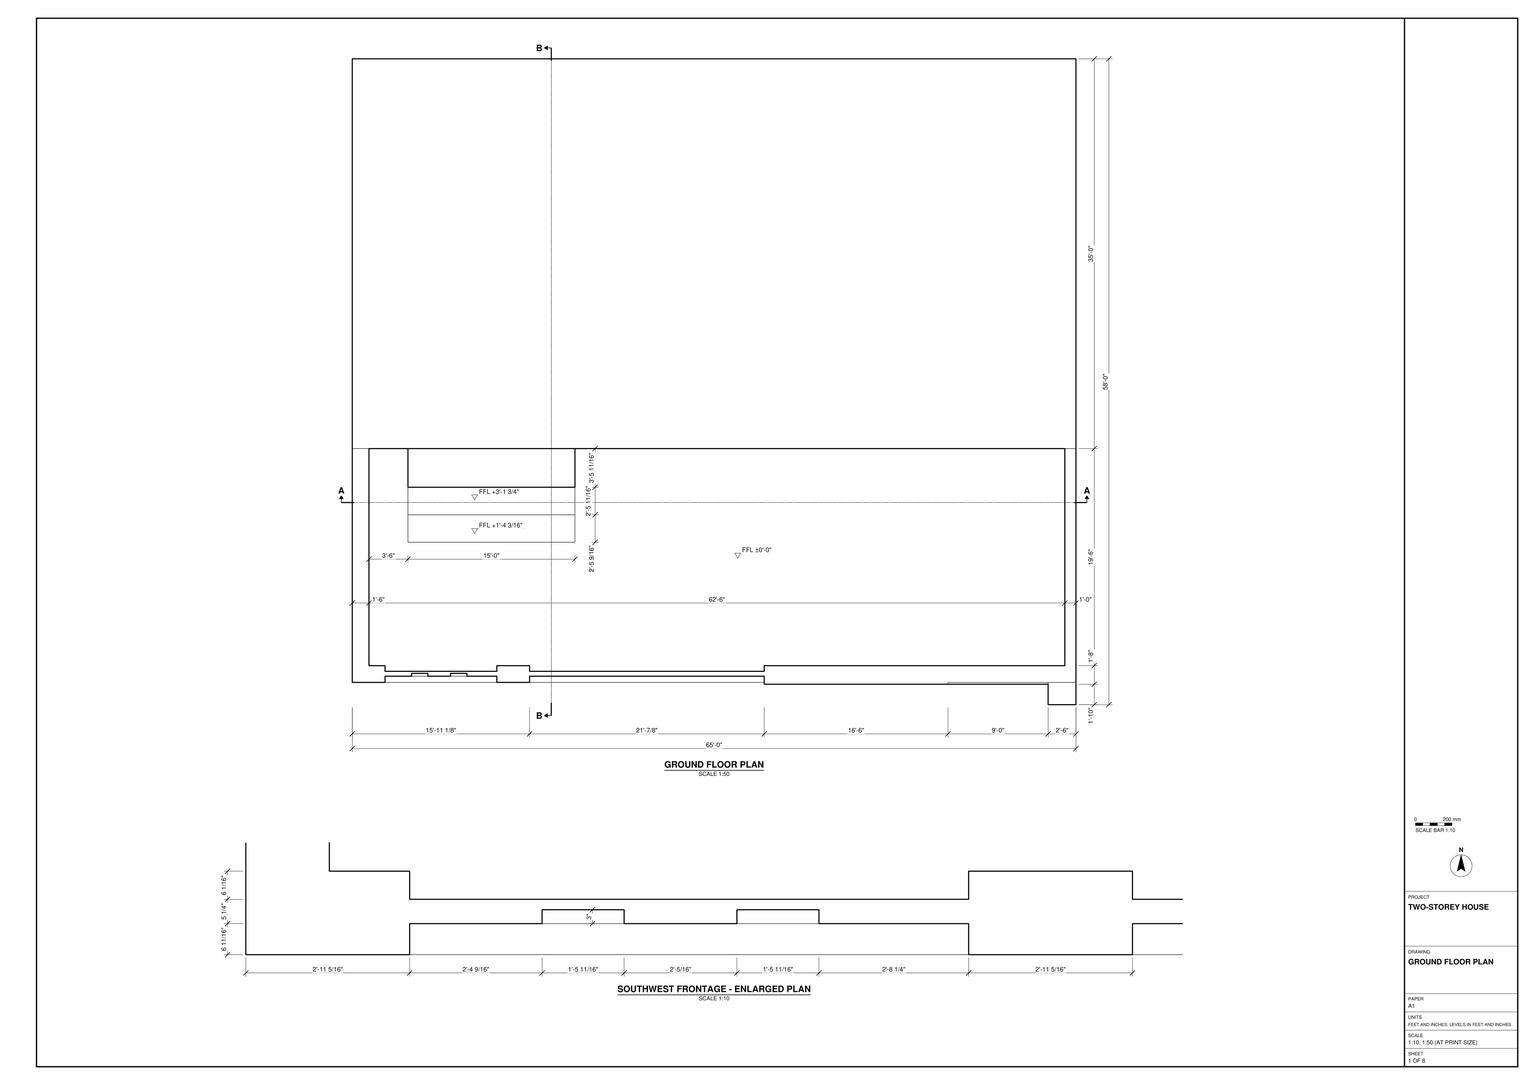
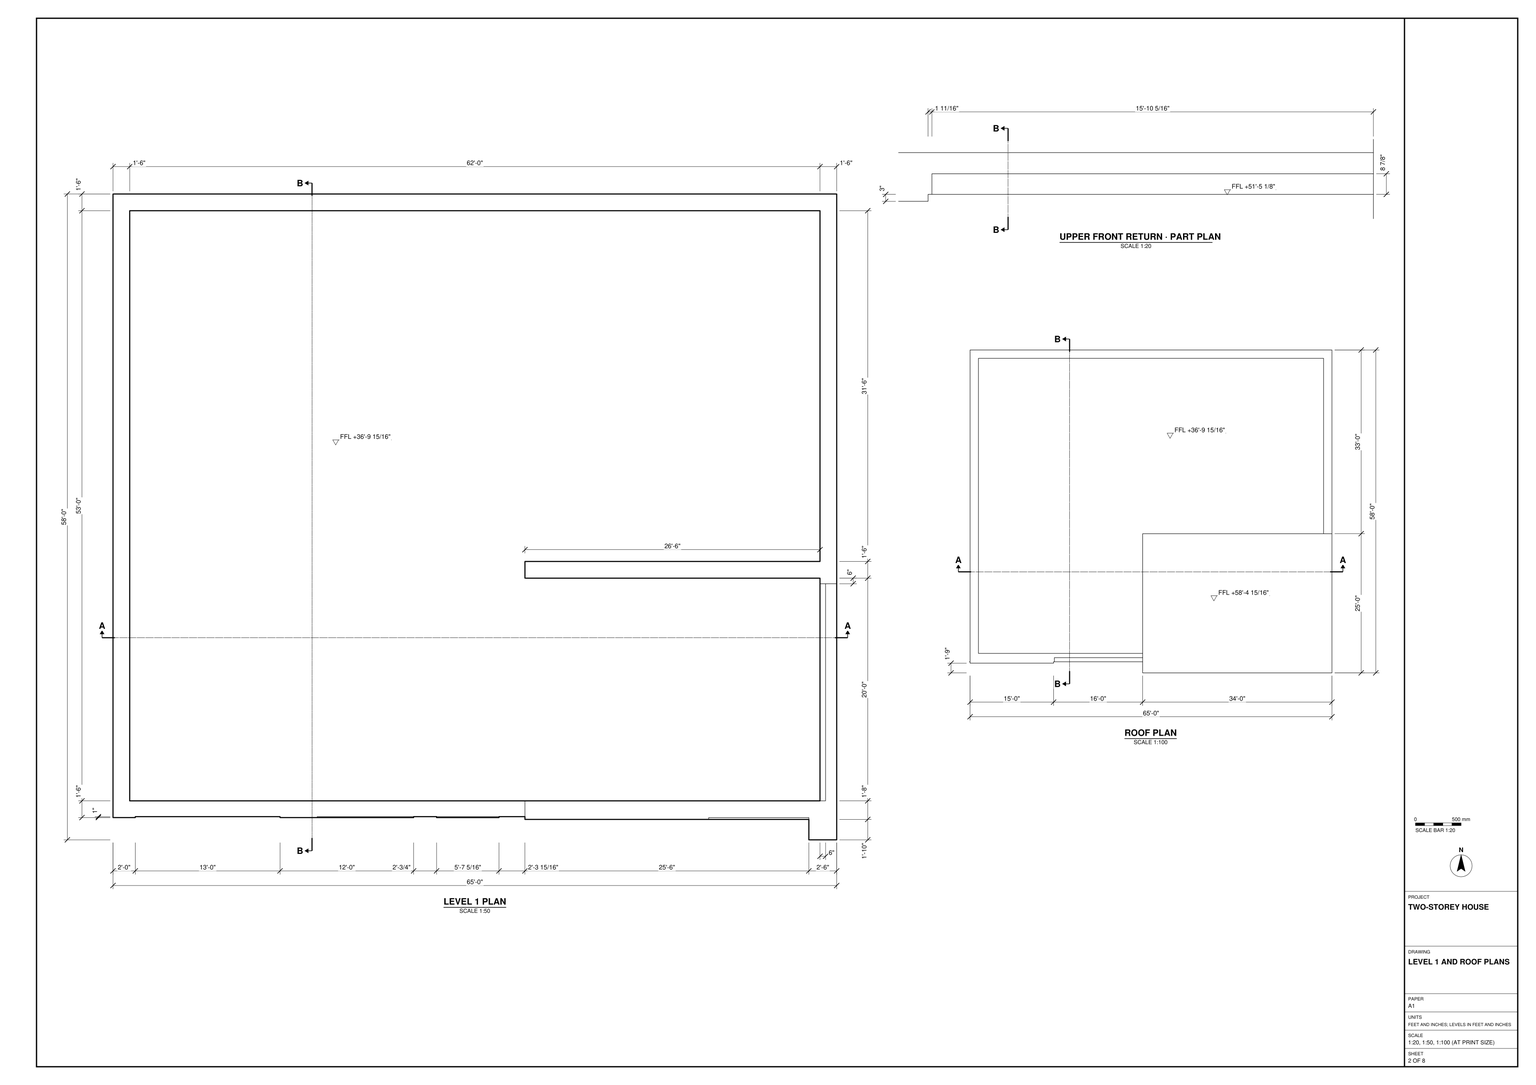
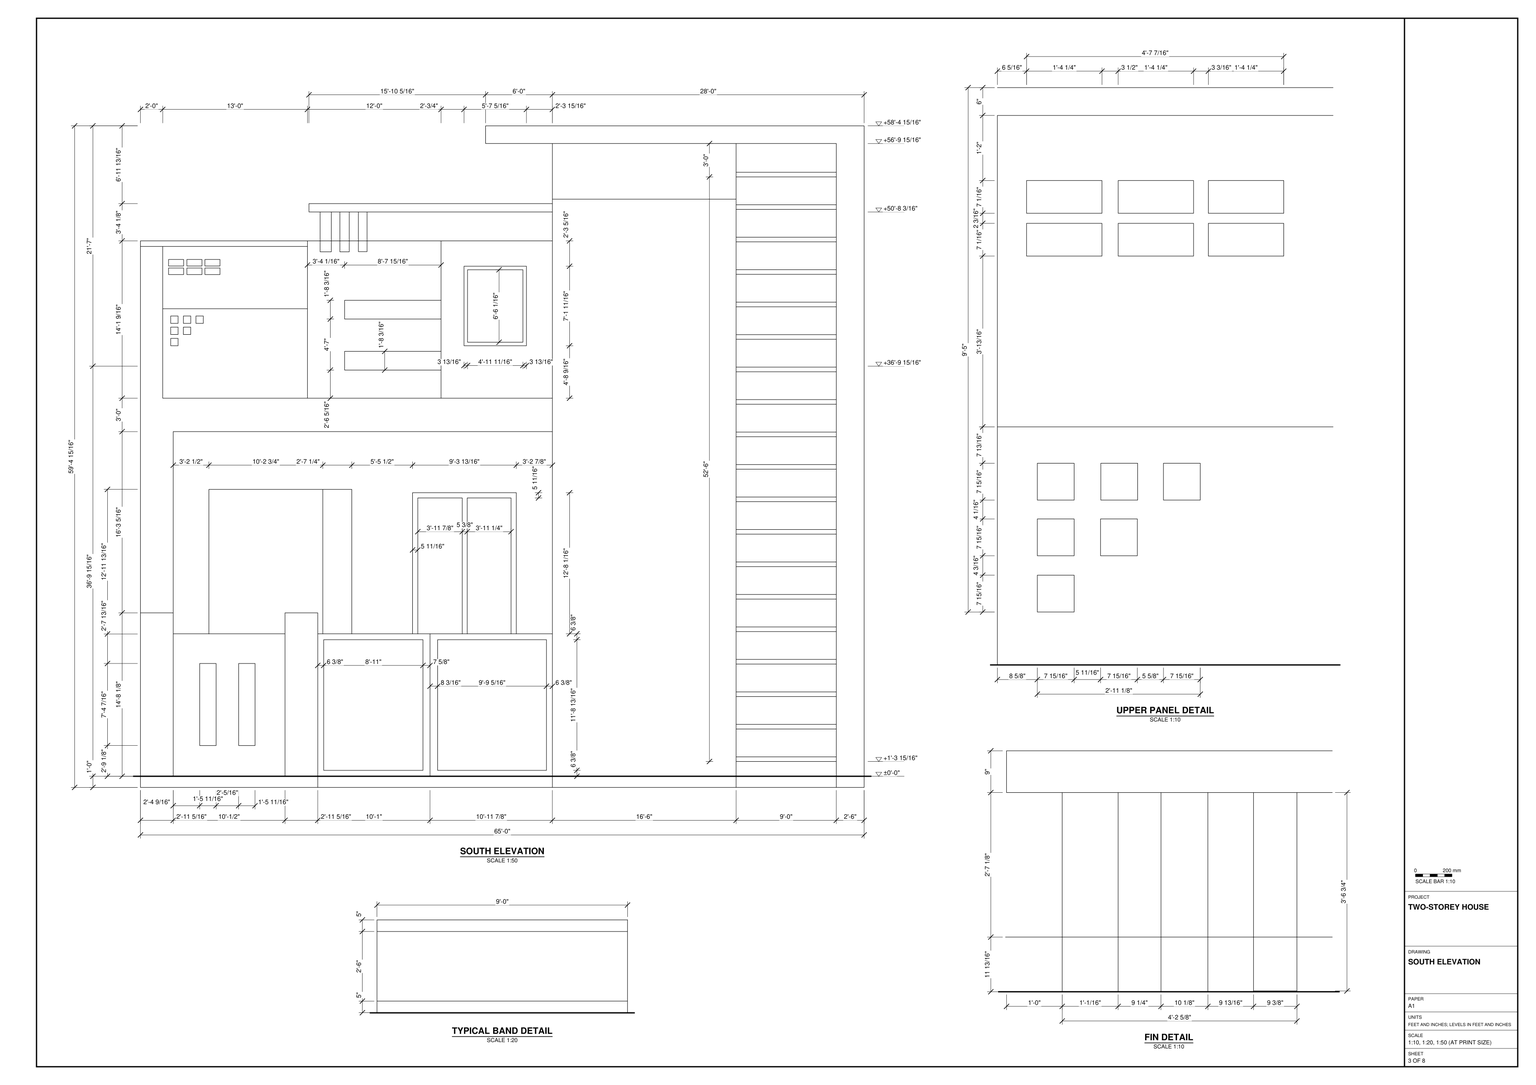
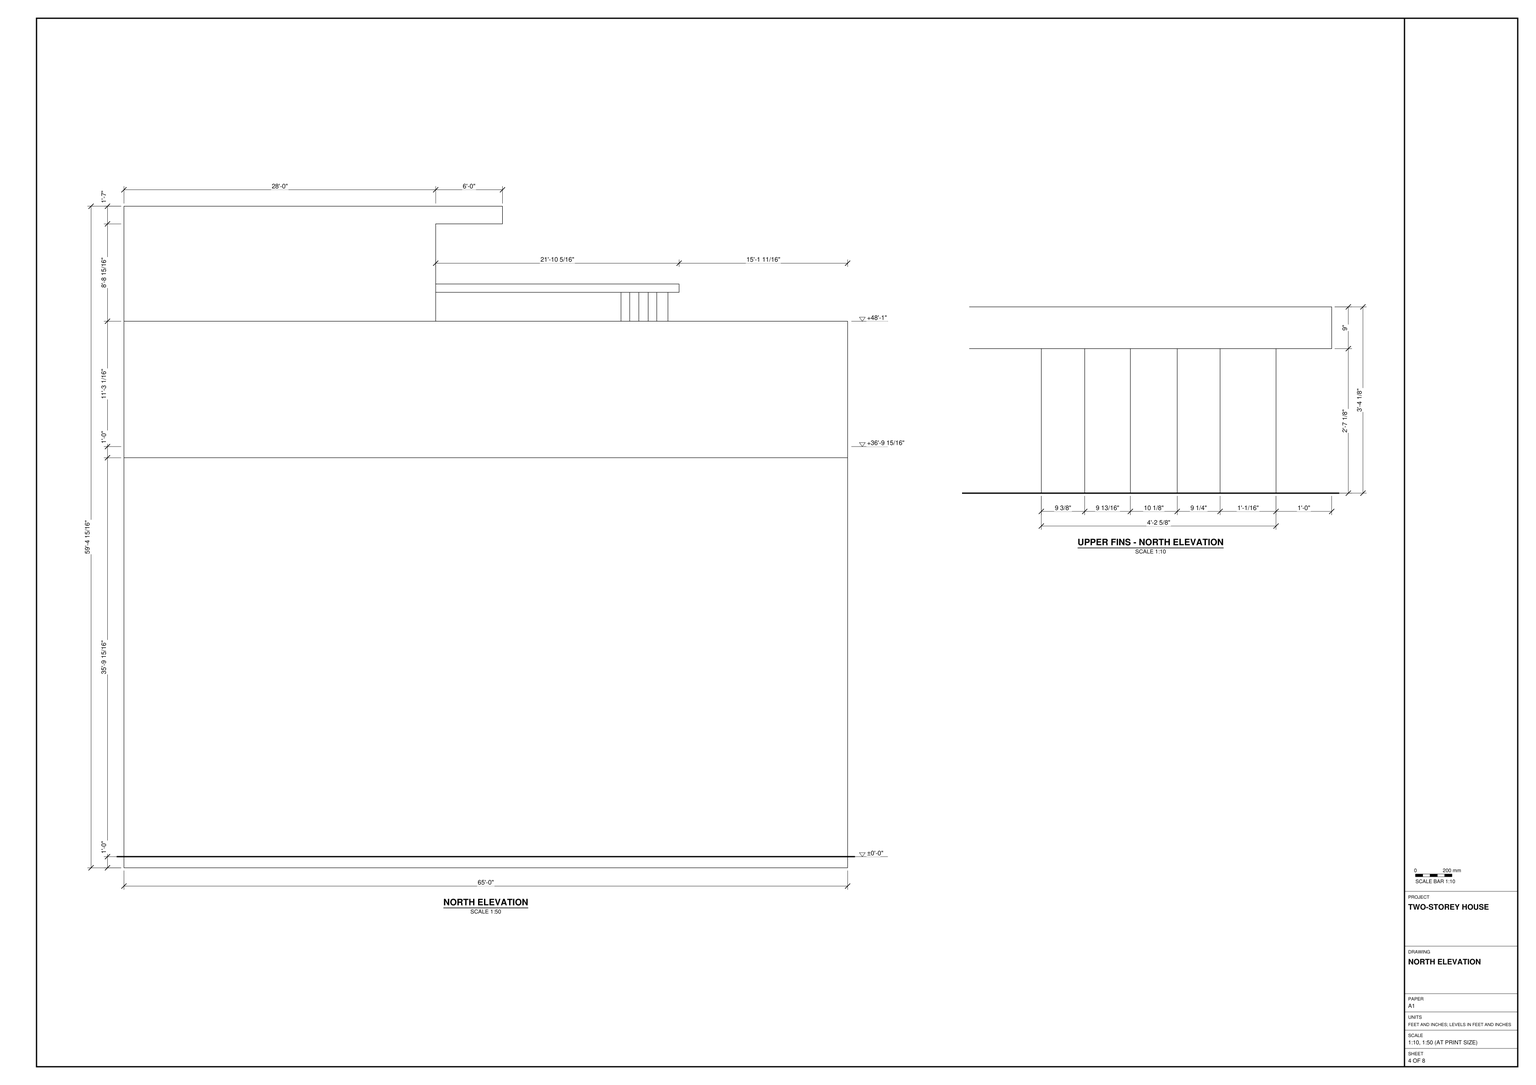
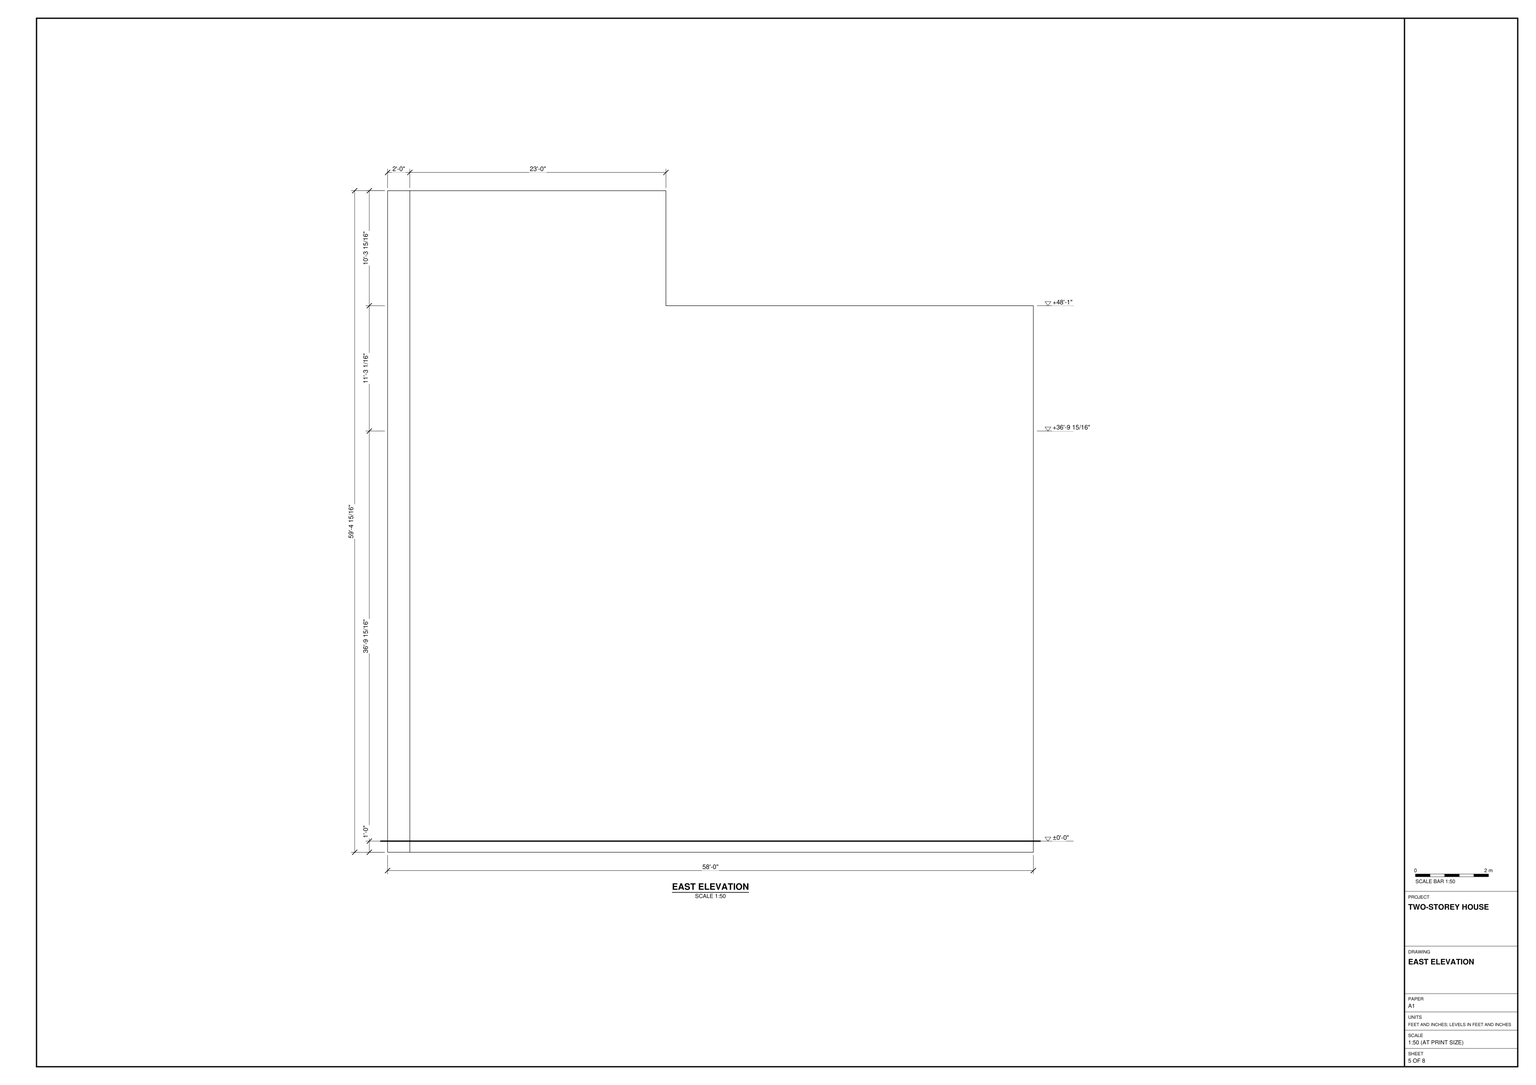
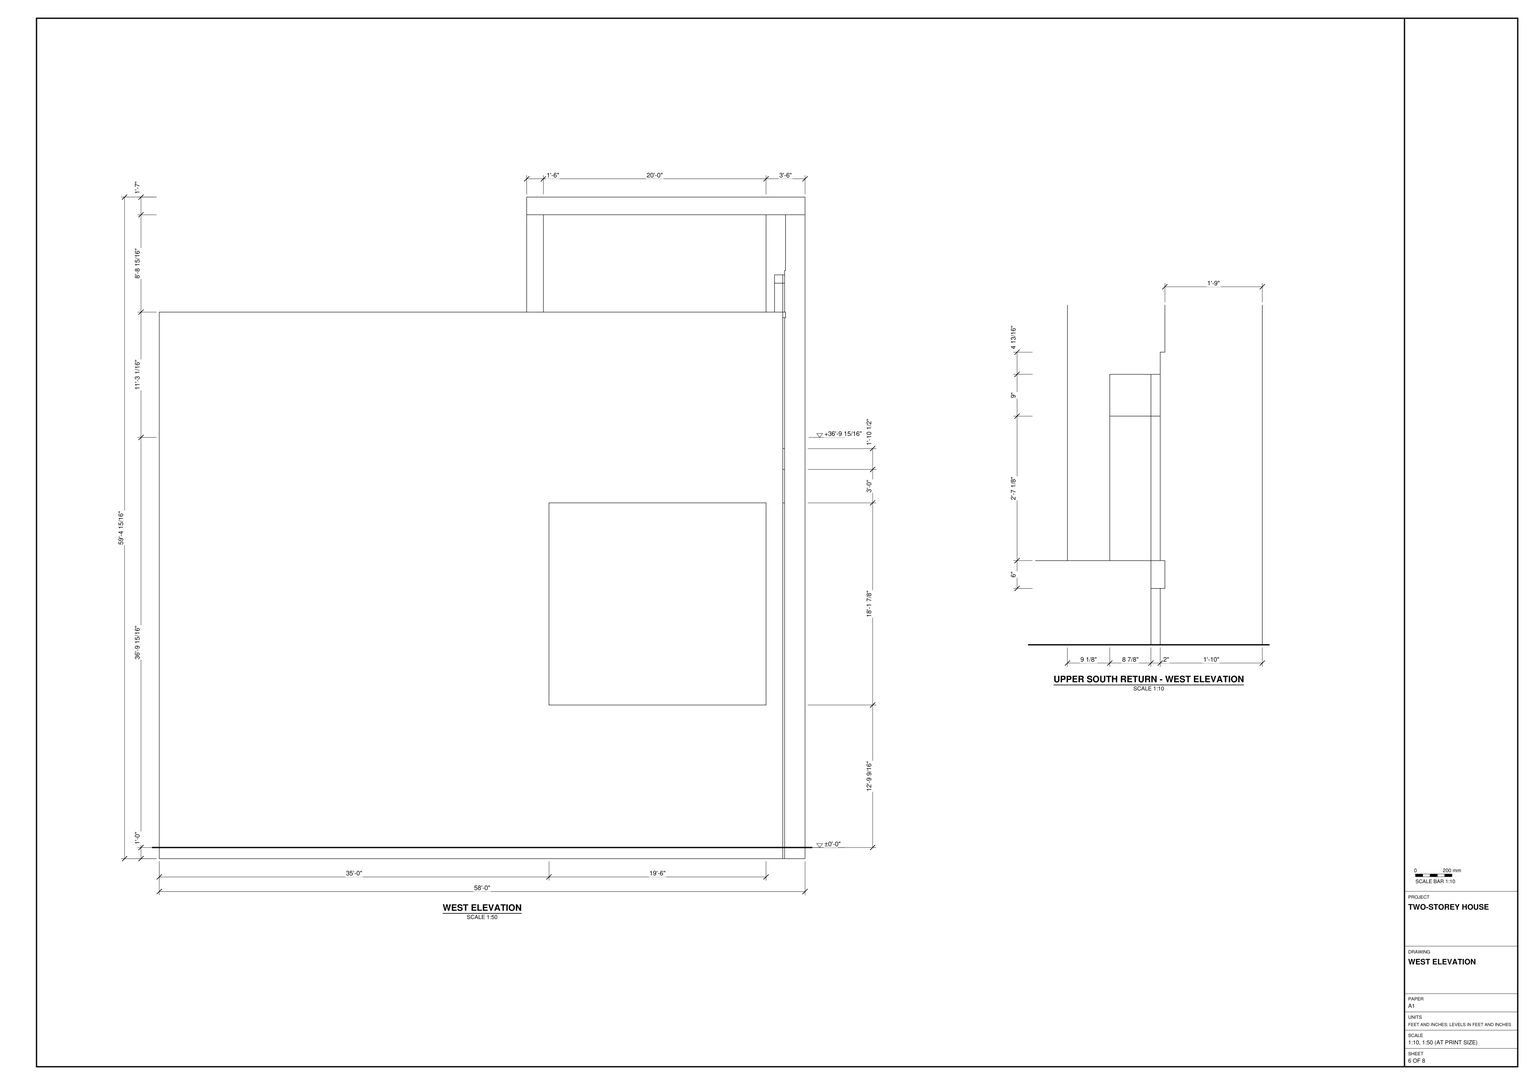
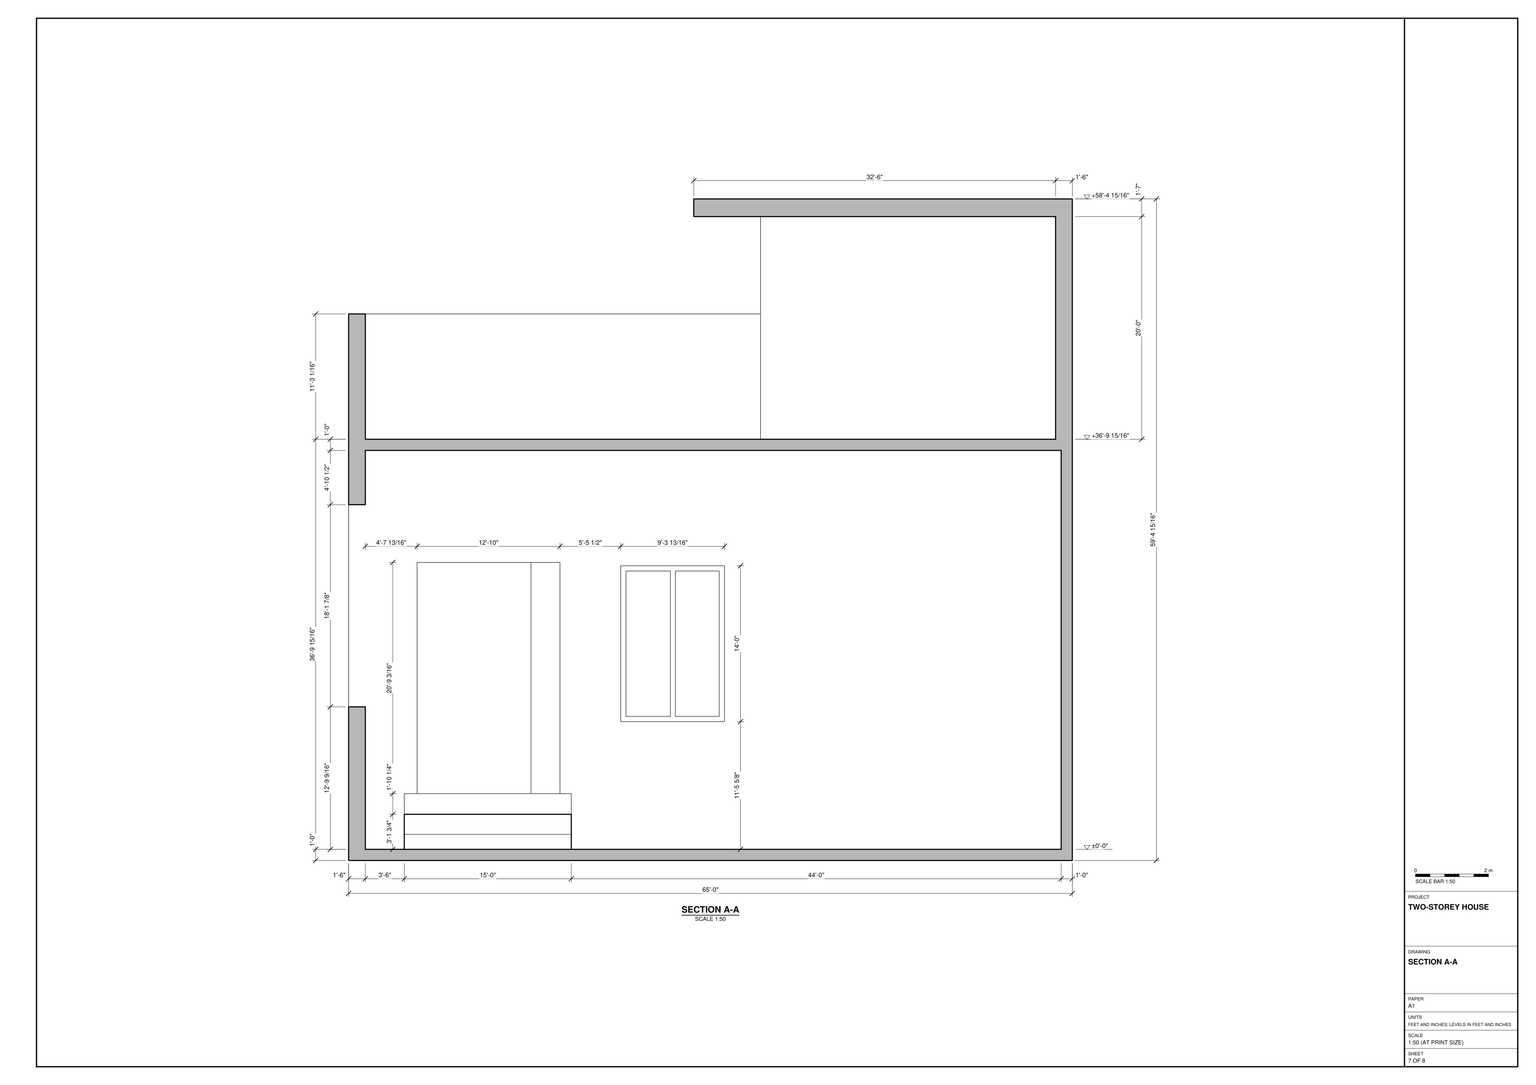
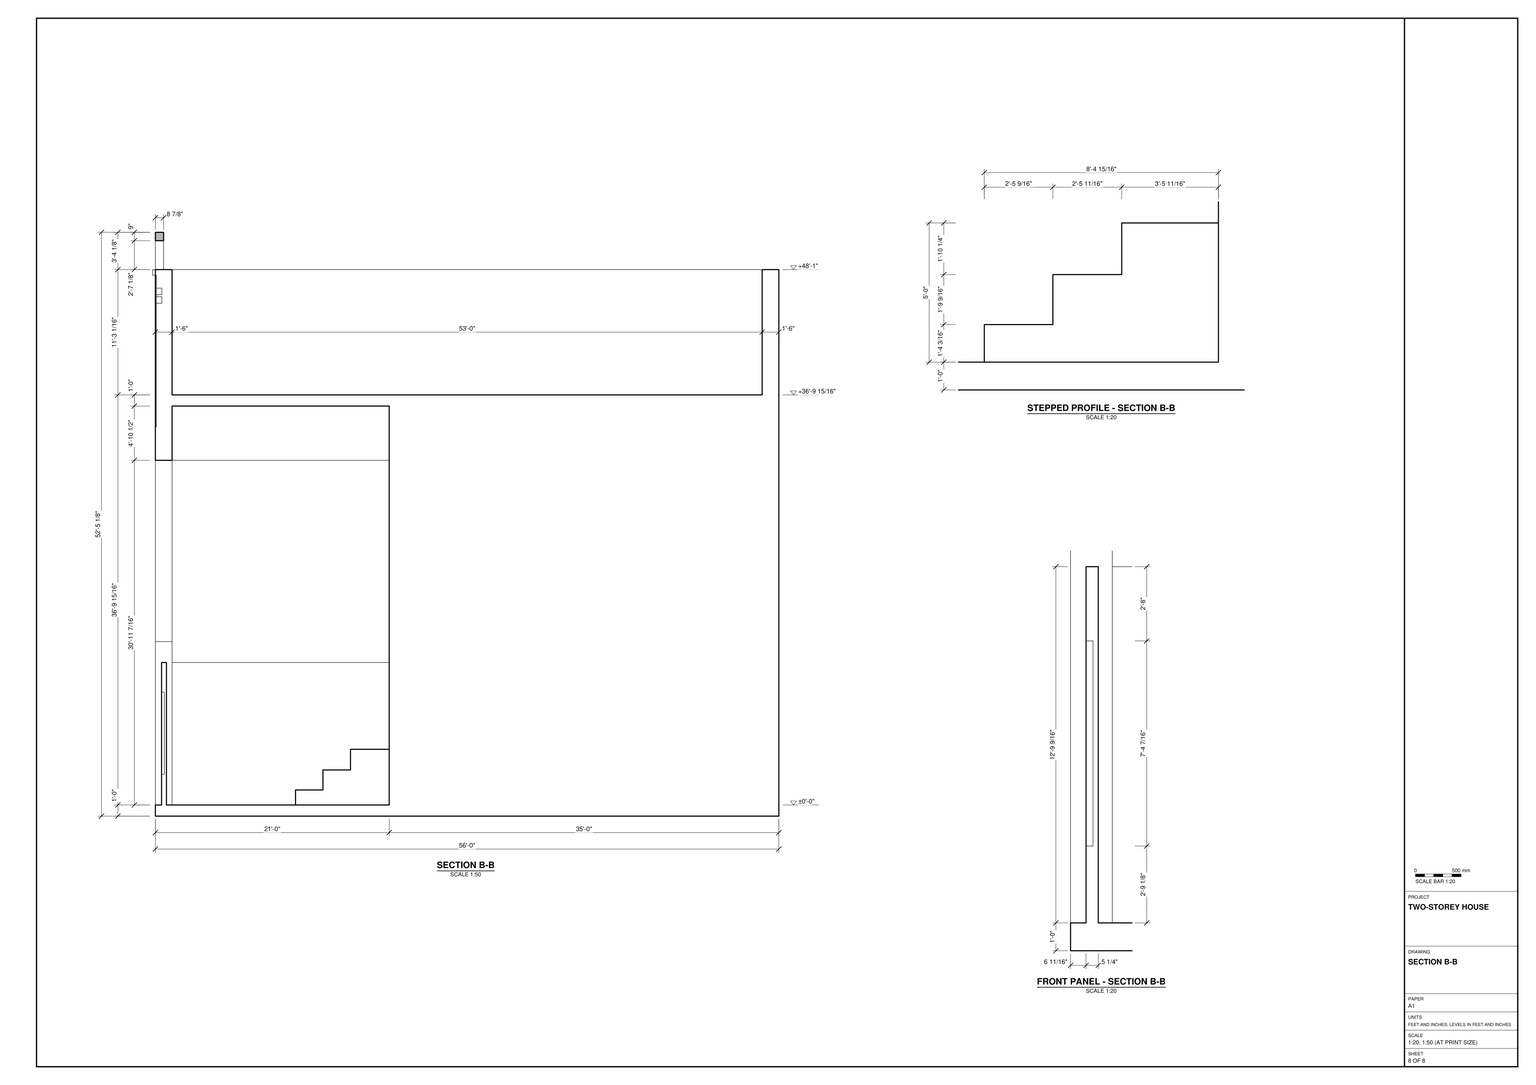
Build the two-storey house in SketchUp from task_files/diagram_01.pdf. Work in feet and inches. Set out the house with the south frontage along the X axis. The overall width is 65'-0", the depth is 58'-0", and the height from the lowest to the highest point is 59'-4 15/16". Use ±0'-0" for the ground floor and +36'-9 15/16" for the upper level.

Follow the plans for the slab edges, wall thicknesses and returns. Include the stepped platform near the left end of the ground-floor space and the wall extending inward from the right side on the upper level. Form the flat roof at the heights shown, with its raised rectangular portion at the southeast corner.

Use the enlarged frontage plan and south elevation together: set the piers, panels and framed openings at their drawn depths rather than placing them all on one plane. Include the small rectangular and square details on the upper left panel, the short fins below the projecting cap, and the horizontal bands on the tall right-hand bay.

Keep the walls, slabs and roof as separate groups or components. Group each furniture or joinery piece separately where shown, and use components for repeated parts. Decor and loose items, if included, may be any suitable library components. Save one SketchUp model as output_files/two_storey_house_with_a_stepped_south_frontage.skp.

# SketchUp Ruby script. Lengths in inches.
U = 1.inch
M = Sketchup.active_model
def pt(a) = Geom::Point3d.new(a.map { |v| v * U })
def face(e, loops, mat)
  f = e.add_face(loops[0].map { |a| pt(a) })
  loops[1..].each { |l| e.add_face(l.map { |a| pt(a) }).erase! }
  f.material = f.back_material = mat if mat
  f
end
# faces: each face lists its corners as indices into pts; further lists are holes
def faces(e, pts, list, mat = nil) = list.each { |f| face(e, (f[0].is_a?(Array) ? f : [f]).map { |l| l.map { |i| pts[i] } }, mat) }
# xy, xz, yz: faces in a plane at the given z, y or x. An outline is a flat list of corners, or four numbers for a rectangle; further outlines are holes
def ring(l) = l.size == 4 ? [[l[0], l[1]], [l[2], l[1]], [l[2], l[3]], [l[0], l[3]]] : l.each_slice(2).to_a
def flat(e, list, mat, &to3) = list.each { |f| face(e, (f[0].is_a?(Array) ? f : [f]).map { |l| ring(l).map { |u, v| to3.(u, v) } }, mat) }
def xy(e, z, list, mat = nil) = flat(e, list, mat) { |x, y| [x, y, z] }
def xz(e, y, list, mat = nil) = flat(e, list, mat) { |x, z| [x, y, z] }
def yz(e, x, list, mat = nil) = flat(e, list, mat) { |y, z| [x, y, z] }
def lines(e, pts, list) = list.each { |a, b| e.add_line(pt(pts[a]), pt(pts[b])) }
# prism: a flat outline (further loops are holes) pulled along v
def prism(e, loops, v, mat = nil)
  f = face(e, loops, mat); d = Geom::Vector3d.new(v.map { |x| x * U })
  f.pushpull(f.normal.samedirection?(d) ? d.length : -d.length)
end
def box(e, o, s, mat = nil) = prism(e, [[o, [o[0] + s[0], o[1], o[2]], [o[0] + s[0], o[1] + s[1], o[2]], [o[0], o[1] + s[1], o[2]]]], [0, 0, s[2]], mat)
def at(x, y, z, deg = 0) = Geom::Transformation.translation(pt([x, y, z])) * Geom::Transformation.rotation(ORIGIN, Z_AXIS, deg.degrees)
def axes(o, x, y, z) = Geom::Transformation.new([*x, 0, *y, 0, *z, 0, *pt(o).to_a, 1])
def part(name) = M.definitions.add(name)
# library, detail: a bought-in or finely detailed component or shape, given as its bounding box
def library(name, o, s) = part(name).tap { |d| box(d.entities, o, s) }
def detail(e, o, s) = box(e.add_group.entities, o, s)
def put(e, d, t, mat = nil) = e.add_instance(d, t).tap { |i| i.material = mat if mat }
def group(e, t, mat = nil) = e.add_group.tap { |g| g.transformation = t; g.material = mat if mat }.entities
root = M.entities
M.materials.add("[0005_LightPink]").color = [255, 182, 193]
M.materials.add("[0012_Bisque]").color = [211, 189, 162]
M.materials.add("[0012_Bisque]1").color = [186, 166, 143]
M.materials.add("[0018_Brown]").color = [71, 18, 18]
M.materials.add("[0026_LightSalmon]").color = [198, 124, 95]
M.materials.add("[0111_SlateGray]").color = [79, 90, 102]
M.materials.add("[0137_Black]").color = [0, 0, 0]
M.materials.add("[Cladding Siding Tan]").color = [119, 93, 70]
M.materials.add("[Granite Brown]").color = [126, 104, 91]
M.materials.add("[Herringbone 4x1]").color = [132, 132, 132]
M.materials.add("[Stone Flagstone Ashlar]").color = [175, 116, 102]
M.materials.add("[Stone Marble]").color = [143, 138, 136]
M.materials.add("[Translucent Glass Gray]").color = [123, 128, 82]
M.materials["[Translucent Glass Gray]"].alpha = 0.5
xy(root,0,[[750,0,780,24],[444,22,444,24,0,24,0,696,780,696,780,24,750,24,750,22]])
xy(root,12,[[60,175.0625,240,196.125],[60,196.125,240,276]])
xy(root,12,[[35.3125,24,155.8125,30.6875]],"[Stone Flagstone Ashlar]")
xy(root,12,[[191.125,24,444,30.6875],[35.3125,35.9375,155.8125,35.9375,155.8125,42,191.125,42,191.125,35.9375,444,35.9375,444,42,768,42,768,276,240,276,240,175.0625,60,175.0625,60,276,18,276,18,42,35.3125,42]],"[Stone Marble]")
xy(root,27.9375,[[642,22,750,24]])
xy(root,28.1875,[[60,175.0625,240,204.625]],"[Granite Brown]")
xy(root,32.9375,[[642,22,750,24]])
xy(root,45.12,[[63.86,30.6875,81.55,33.6875],[105.86,30.6875,123.55,33.6875]],"[0012_Bisque]1")
xy(root,49.75,[[60,204.625,240,234.3125]],"[Granite Brown]")
xy(root,62.9375,[[642,22,750,24]])
xy(root,67.9375,[[642,22,750,24]])
xy(root,72,[[60,234.3125,240,276]],"[Granite Brown]")
xy(root,97.9375,[[642,22,750,24]])
xy(root,102.9375,[[642,22,750,24]])
xy(root,132.9375,[[642,22,750,24]])
xy(root,133.55,[[63.86,30.6875,81.55,33.6875],[105.86,30.6875,123.55,33.6875]],"[0012_Bisque]1")
xy(root,137.9375,[[642,22,750,24]])
xy(root,165.5625,[[35.3125,30.6875,155.8125,35.9375],[191.125,30.6875,444,35.9375]])
xy(root,165.5625,[[0,42,18,276]],"[0111_SlateGray]")
xy(root,167.9375,[[642,22,750,24]])
xy(root,172.9375,[[642,22,750,24]])
xy(root,188.125,[[155.8125,24,191.125,42]],"[Stone Flagstone Ashlar]")
xy(root,202.9375,[[642,22,750,24]])
xy(root,207.9375,[[642,22,750,24]])
xy(root,237.9375,[[642,22,750,24]])
xy(root,242.9375,[[642,22,750,24]])
xy(root,272.9375,[[642,22,750,24]])
xy(root,277.9375,[[642,22,750,24]])
xy(root,307.9375,[[642,22,750,24]])
xy(root,312.9375,[[642,22,750,24]])
xy(root,342.9375,[[642,22,750,24]])
xy(root,347.9375,[[642,22,750,24]])
xy(root,377.9375,[[642,22,750,24]])
xy(root,382.9375,[[642,22,750,24]])
xy(root,383.4375,[[35.3125,24,444,42],[0,42,18,276]],"[0012_Bisque]")
xy(root,412.9375,[[642,22,750,24]])
xy(root,417.9375,[[642,22,750,24]])
xy(root,419.4375,[[24,24,180,25],[324,24,444,25]])
xy(root,441.9375,[[18,42,768,276]],"[0012_Bisque]")
xy(root,447.9375,[[642,22,750,24]])
xy(root,449.76,[[220.0625,24,324,25]])
xy(root,452.9375,[[642,22,750,24]])
xy(root,453.9375,[[18,42,762,42,762,282,444,282,444,300,762,300,762,678,18,678]])
xy(root,469.94,[[220.0625,24,324,25]])
xy(root,475.98,[[348.73,24,416.04,25]])
xy(root,482.9375,[[642,22,750,24]])
xy(root,487.9375,[[642,22,750,24]])
xy(root,504.76,[[220.0625,24,324,25]])
xy(root,517.9375,[[642,22,750,24]])
xy(root,522.9375,[[642,22,750,24]])
xy(root,524.94,[[220.0625,24,324,25]])
xy(root,552.6875,[[30.3,25,46.55,31],[50.05,25,66.3,31],[69.49,25,85.74,31]],"[0012_Bisque]")
xy(root,552.9375,[[642,22,750,24]])
xy(root,557.9375,[[642,22,750,24]])
xy(root,559.75,[[30.3,25,46.55,31],[50.05,25,66.3,31],[69.49,25,85.74,31]],"[0012_Bisque]")
xy(root,561.67,[[348.73,24,416.04,25]])
xy(root,561.91,[[30.3,25,46.55,31],[50.05,25,66.3,31],[69.49,25,85.74,31]],"[0012_Bisque]")
xy(root,568.98,[[30.3,25,46.55,31],[50.05,25,66.3,31],[69.49,25,85.74,31]],"[0012_Bisque]")
xy(root,583,[[0,21,0,24,24,24,24,25,180,25,180,21]])
xy(root,587.9375,[[642,22,750,24]])
xy(root,589,[[0,21,180,21,180,24,193.66,24,193.66,32.875,205.72,32.875,205.72,24,214.96,24,214.96,32.875,225.06,32.875,225.06,24,234.9,24,234.9,32.875,244.25,32.875,244.25,24,324,24,324,25,444,25,444,42,18,42,18,678,762,678,762,300,780,300,780,696,0,696],[193.66,24,205.72,32.875],[214.96,24,225.06,32.875],[234.9,24,244.25,32.875]])
xy(root,592.9375,[[642,22,750,24]])
xy(root,620.15,[[181.66,24,193.66,32.875],[193.66,24,205.72,32.875],[205.72,24,214.96,32.875],[214.96,24,225.06,32.875],[225.06,24,234.9,32.875],
  [234.9,24,244.25,32.875],[244.25,24,444,32.875]])
xy(root,622.9375,[[642,22,750,24]])
xy(root,627.9375,[[642,22,750,24]])
xy(root,629.15,[[181.66,24,444,32.875]])
xy(root,633.9375,[[444,21,642,22]])
xy(root,657.9375,[[642,22,750,24]])
xy(root,662.9375,[[642,22,750,24]])
xy(root,693.9375,[[472.15,8.13,471.37,8.22,470.64,8.5,470.01,8.97,469.52,9.58,469.21,10.3,469.09,11.07,469.18,11.85,469.47,12.58,469.93,13.21,470.55,13.7,471.26,14.01,472.04,14.125,472.82,14.04,473.54,13.75,474.17,13.29,474.66,12.67,474.98,11.96,475.09,11.18,475,10.4,474.72,9.67,474.25,9.04,473.64,8.56,472.92,8.24],[546.65,8.13,545.87,8.22,545.14,8.5,544.51,8.97,544.02,9.58,543.71,10.3,543.59,11.07,543.68,11.85,543.97,12.58,544.43,13.21,545.05,13.7,545.76,14.01,546.54,14.125,547.32,14.04,548.04,13.75,548.67,13.29,549.16,12.67,549.48,11.96,549.59,11.18,549.5,10.4,549.22,9.67,548.75,9.04,548.14,8.56,547.42,8.24],[631.77,8.13,630.99,8.22,630.26,8.5,629.63,8.97,629.15,9.58,628.83,10.3,628.72,11.07,628.81,11.85,629.09,12.58,629.56,13.21,630.17,13.7,630.89,14.01,631.66,14.125,632.44,14.04,633.17,13.75,633.8,13.29,634.29,12.67,634.6,11.96,634.72,11.18,634.63,10.4,634.34,9.67,633.875,9.04,633.26,8.56,632.55,8.24],[715.9,8.13,715.12,8.22,714.39,8.5,713.76,8.97,713.27,9.58,712.96,10.3,712.84,11.07,712.93,11.85,713.22,12.58,713.68,13.21,714.3,13.7,715.01,14.01,715.79,14.125,716.57,14.04,717.29,13.75,717.92,13.29,718.41,12.67,718.73,11.96,718.84,11.18,718.75,10.4,718.47,9.67,718,9.04,717.39,8.56,716.67,8.24],[405.375,37.23,403.82,37.39,402.35,37.95,401.09,38.87,400.1,40.09,399.46,41.52,399.21,43.0625,399.375,44.62,399.9375,46.09,400.86,47.35,402.07,48.34,403.5,48.98,405.05,49.23,406.61,49.0625,408.07,48.5,409.34,47.58,410.32,46.37,410.96,44.9375,411.21,43.39,411.05,41.83,410.49,40.37,409.57,39.1,408.35,38.11,406.92,37.48],
  [405.375,125.67,403.82,125.83,402.35,126.39,401.09,127.31,400.1,128.52,399.46,129.95,399.21,131.5,399.375,133.06,399.9375,134.52,400.86,135.79,402.07,136.78,403.5,137.42,405.05,137.66,406.61,137.5,408.07,136.94,409.34,136.02,410.32,134.81,410.96,133.375,411.21,131.83,411.05,130.27,410.49,128.81,409.57,127.54,408.35,126.55,406.92,125.91],[405.375,218.17,403.82,218.33,402.35,218.89,401.09,219.81,400.1,221.02,399.46,222.45,399.21,224,399.375,225.56,399.9375,227.02,400.86,228.29,402.07,229.28,403.5,229.92,405.05,230.16,406.61,230,408.07,229.44,409.34,228.52,410.32,227.31,410.96,225.875,411.21,224.33,411.05,222.77,410.49,221.31,409.57,220.04,408.35,219.05,406.92,218.41]])
xy(root,693.9375,[[[372,0,372,300,444,300,444,282,762,282,762,42,444,42,444,21,642,21,642,22,750,22,750,0],[405.375,125.67,406.92,125.91,408.35,126.55,409.57,127.54,410.49,128.81,411.05,130.27,411.21,131.83,410.96,133.375,410.32,134.81,409.34,136.02,408.07,136.94,406.61,137.5,405.05,137.66,403.5,137.42,402.07,136.78,400.86,135.79,399.9375,134.52,399.375,133.06,399.21,131.5,399.46,129.95,400.1,128.52,401.09,127.31,402.35,126.39,403.82,125.83],[405.375,218.17,406.92,218.41,408.35,219.05,409.57,220.04,410.49,221.31,411.05,222.77,411.21,224.33,410.96,225.875,410.32,227.31,409.34,228.52,408.07,229.44,406.61,230,405.05,230.16,403.5,229.92,402.07,229.28,400.86,228.29,399.9375,227.02,399.375,225.56,399.21,224,399.46,222.45,400.1,221.02,401.09,219.81,402.35,218.89,403.82,218.33],[405.375,37.23,406.92,37.48,408.35,38.11,409.57,39.1,410.49,40.37,411.05,41.83,411.21,43.39,410.96,44.9375,410.32,46.37,409.34,47.58,408.07,48.5,406.61,49.0625,405.05,49.23,403.5,48.98,402.07,48.34,400.86,47.35,399.9375,46.09,399.375,44.62,399.21,43.0625,399.46,41.52,400.1,40.09,401.09,38.87,402.35,37.95,403.82,37.39],[472.15,8.13,472.92,8.24,473.64,8.56,474.25,9.04,474.72,9.67,475,10.4,475.09,11.18,474.98,11.96,474.66,12.67,474.17,13.29,473.54,13.75,472.82,14.04,472.04,14.125,471.26,14.01,470.55,13.7,469.93,13.21,469.47,12.58,469.18,11.85,469.09,11.07,469.21,10.3,469.52,9.58,470.01,8.97,470.64,8.5,471.37,8.22],[546.65,8.13,547.42,8.24,548.14,8.56,548.75,9.04,549.22,9.67,549.5,10.4,549.59,11.18,549.48,11.96,549.16,12.67,548.67,13.29,548.04,13.75,547.32,14.04,546.54,14.125,545.76,14.01,545.05,13.7,544.43,13.21,543.97,12.58,543.68,11.85,543.59,11.07,543.71,10.3,544.02,9.58,544.51,8.97,545.14,8.5,545.87,8.22],[631.77,8.13,632.55,8.24,633.26,8.56,633.875,9.04,634.34,9.67,634.63,10.4,634.72,11.18,634.6,11.96,634.29,12.67,633.8,13.29,633.17,13.75,632.44,14.04,631.66,14.125,630.89,14.01,630.17,13.7,629.56,13.21,629.09,12.58,628.81,11.85,628.72,11.07,628.83,10.3,629.15,9.58,629.63,8.97,630.26,8.5,630.99,8.22],[715.9,8.13,716.67,8.24,717.39,8.56,718,9.04,718.47,9.67,718.75,10.4,718.84,11.18,718.73,11.96,718.41,12.67,717.92,13.29,717.29,13.75,716.57,14.04,715.79,14.125,715.01,14.01,714.3,13.7,713.68,13.21,713.22,12.58,712.93,11.85,712.84,11.07,712.96,10.3,713.27,9.58,713.76,8.97,714.39,8.5,715.12,8.22]]],"[0012_Bisque]")
xy(root,712.9375,[[372,0,780,300]])
xz(root,0,[[750,0,780,0,780,712.9375,372,712.9375,372,693.9375,750,693.9375]],"[0012_Bisque]")
xz(root,21,[[0,583,180,589]])
xz(root,21,[[444,633.9375,642,693.9375]],"[0012_Bisque]")
xz(root,22,[[444,0,642,633.9375]],"[Herringbone 4x1]")
xz(root,22,[[642,0,750,27.9375],[642,32.9375,750,62.9375],[642,67.9375,750,97.9375],[642,102.9375,750,132.9375],[642,137.9375,750,167.9375],
  [642,172.9375,750,202.9375],[642,207.9375,750,237.9375],[642,242.9375,750,272.9375],[642,277.9375,750,307.9375],[642,312.9375,750,342.9375],
  [642,347.9375,750,377.9375],[642,382.9375,750,412.9375],[642,417.9375,750,447.9375],[642,452.9375,750,482.9375],[642,487.9375,750,517.9375],
  [642,522.9375,750,552.9375],[642,557.9375,750,587.9375],[642,592.9375,750,622.9375],[642,627.9375,750,657.9375],[642,662.9375,750,693.9375]],"[Stone Flagstone Ashlar]")
xz(root,24,[[642,27.9375,750,32.9375],[642,62.9375,750,67.9375],[642,97.9375,750,102.9375],[642,132.9375,750,137.9375],[642,167.9375,750,172.9375],
  [642,202.9375,750,207.9375],[642,237.9375,750,242.9375],[642,272.9375,750,277.9375],[642,307.9375,750,312.9375],[642,342.9375,750,347.9375],
  [642,377.9375,750,382.9375],[642,412.9375,750,417.9375],[642,447.9375,750,452.9375],[[348.73,475.98,416.04,561.67],[352.54,479.79,412.23,557.86]],[352.54,479.79,412.23,557.86],
  [642,482.9375,750,487.9375],[642,517.9375,750,522.9375],[642,552.9375,750,557.9375],[193.66,577.21,205.72,589],[214.96,577.21,225.06,589],
  [234.9,577.39,244.25,589],[642,587.9375,750,592.9375],[193.66,589,205.72,620.15],[214.96,589,225.06,620.15],[234.9,589,244.25,620.15],
  [181.66,620.15,444,629.15],[642,622.9375,750,627.9375],[642,657.9375,750,662.9375]])
xz(root,24,[[180,419.4375,324,419.4375,324,449.76,220.0625,449.76,220.0625,469.94,324,469.94,324,504.76,220.0625,504.76,220.0625,524.94,324,524.94,324,589,244.25,589,244.25,577.39,234.9,577.39,234.9,589,225.06,589,225.06,577.21,214.96,577.21,214.96,589,205.72,589,205.72,577.21,193.66,577.21,193.66,589,180,589]],"[0012_Bisque]")
xz(root,24,[[0,188.125,35.3125,188.125,35.3125,383.4375,444,383.4375,444,419.4375,24,419.4375,24,583,0,583]],"[0111_SlateGray]")
xz(root,24,[[0,0,191.125,0,191.125,188.125,155.8125,188.125,155.8125,12,0,12],[0,12,35.3125,188.125]],"[Stone Flagstone Ashlar]")
xz(root,24,[[191.125,0,444,12]],"[Stone Marble]")
xz(root,25,[[32.62,475.97,40.56,483.91],[32.62,488.1,40.56,496.04],[46.24,488.1,54.18,496.04],[32.62,500.1,40.56,508.04],[46.31,500.1,54.24,508.04],
  [59.81,500.1,67.74,508.04]])
xz(root,25,[[[24,419.4375,180,515.875],[32.62,500.1,40.56,508.04],[46.31,500.1,54.24,508.04],[59.81,500.1,67.74,508.04],[32.62,488.1,40.56,496.04],[46.24,488.1,54.18,496.04],[32.62,475.97,40.56,483.91]],[[324,419.4375,444,589],[348.73,475.98,416.04,561.67]],[[24,515.875,180,583],[30.3,561.91,46.55,568.98],[50.05,561.91,66.3,568.98],[69.49,561.91,85.74,568.98],[30.3,552.6875,46.55,559.75],[50.05,552.6875,66.3,559.75],[69.49,552.6875,85.74,559.75]]],"[0005_LightPink]")
xz(root,25,[[220.0625,449.76,324,469.94],[220.0625,504.76,324,524.94]],"[0026_LightSalmon]")
xz(root,30.6875,[[[191.125,12,312.125,165.5625],[197.5,18.38,304.5,159.19]],[[312.125,12,444,165.5625],[320.31,18.38,437.62,159.19]]],"[0137_Black]")
xz(root,30.6875,[[197.5,18.38,304.5,159.19],[320.31,18.38,437.62,159.19]],"[Cladding Siding Tan]")
xz(root,30.6875,[[[35.3125,12,155.8125,165.5625],[63.86,45.12,81.55,133.55],[105.86,45.12,123.55,133.55]]],"[Stone Flagstone Ashlar]")
xz(root,31,[[30.3,552.6875,46.55,559.75],[50.05,552.6875,66.3,559.75],[69.49,552.6875,85.74,559.75],[30.3,561.91,46.55,568.98],[50.05,561.91,66.3,568.98],
  [69.49,561.91,85.74,568.98]],"[0012_Bisque]")
xz(root,32.875,[[193.66,589,205.72,620.15],[214.96,589,225.06,620.15],[234.9,589,244.25,620.15],[181.66,620.15,444,629.15]])
xz(root,33.6875,[[63.86,45.12,81.55,133.55],[105.86,45.12,123.55,133.55]],"[0012_Bisque]1")
xz(root,35.9375,[[191.125,12,444,165.5625]])
xz(root,35.9375,[[35.3125,12,155.8125,165.5625]],"[Stone Flagstone Ashlar]")
xz(root,42,[[18,12,18,165.5625,0,165.5625,0,383.4375,35.3125,383.4375,35.3125,12],[18,453.9375,444,589]])
xz(root,42,[[444,12,768,441.9375],[18,383.4375,444,441.9375],[444,453.9375,762,693.9375]],"[0012_Bisque]")
xz(root,42,[[155.8125,12,191.125,188.125]],"[Stone Flagstone Ashlar]")
xz(root,175.0625,[[60,12,240,28.1875]],"[Granite Brown]")
xz(root,204.625,[[60,28.1875,240,49.75]],"[Granite Brown]")
xz(root,234.3125,[[60,49.75,240,72]],"[Granite Brown]")
xz(root,276,[[60,12,240,28.1875],[60,28.1875,240,49.75],[60,49.75,240,72]])
xz(root,276,[[[18,12,60,12,60,72,73.8,72,73.8,321.18,227.8,321.18,227.8,72,240,72,240,12,768,12,768,441.9375,18,441.9375,18,383.4375,0,383.4375,0,165.5625,18,165.5625],[293.29,149.61,405.1,317.61]]],"[0012_Bisque]")
xz(root,276,[[73.8,72,196.55,321.18]],"[0018_Brown]")
xz(root,276,[[[293.29,149.61,405.1,317.61],[298.95,155.28,346.82,311.95],[352.19,155.28,399.4375,311.95]]],"[0137_Black]")
xz(root,276,[[196.55,72,227.8,321.18],[298.95,155.28,346.82,311.95],[352.19,155.28,399.4375,311.95]],"[Translucent Glass Gray]")
xz(root,282,[[444,453.9375,762,693.9375]],"[0012_Bisque]")
xz(root,300,[[444,453.9375,444,693.9375,372,693.9375,372,712.9375,780,712.9375,780,589,762,589,762,453.9375]])
xz(root,678,[[18,453.9375,762,589]])
xz(root,696,[[0,0,780,12],[0,12,780,441.9375],[0,441.9375,780,589]])
yz(root,0,[[[24,0,696,589],[42,165.5625,276,383.4375]],[21,583,24,589]])
yz(root,18,[[42,453.9375,678,589]])
yz(root,18,[[42,383.4375,276,441.9375]],"[0012_Bisque]")
yz(root,18,[[42,12,276,165.5625]],"[0111_SlateGray]")
yz(root,24,[[24,419.4375,25,583]])
yz(root,30.3,[[25,552.6875,31,559.75],[25,561.91,31,568.98]],"[0012_Bisque]")
yz(root,35.3125,[[24,12,30.6875,12,30.6875,165.5625,35.9375,165.5625,35.9375,12,42,12,42,383.4375,24,383.4375]],"[Stone Flagstone Ashlar]")
yz(root,46.55,[[25,552.6875,31,559.75],[25,561.91,31,568.98]],"[0012_Bisque]")
yz(root,50.05,[[25,552.6875,31,559.75],[25,561.91,31,568.98]],"[0012_Bisque]")
yz(root,60,[[175.0625,12,175.0625,28.1875,204.625,28.1875,204.625,49.75,234.3125,49.75,234.3125,72,276,72,276,12]],"[Granite Brown]")
yz(root,63.86,[[30.6875,45.12,33.6875,133.55]],"[0012_Bisque]1")
yz(root,66.3,[[25,552.6875,31,559.75],[25,561.91,31,568.98]],"[0012_Bisque]")
yz(root,69.49,[[25,552.6875,31,559.75],[25,561.91,31,568.98]],"[0012_Bisque]")
yz(root,81.55,[[30.6875,45.12,33.6875,133.55]],"[0012_Bisque]1")
yz(root,85.74,[[25,552.6875,31,559.75],[25,561.91,31,568.98]],"[0012_Bisque]")
yz(root,105.86,[[30.6875,45.12,33.6875,133.55]],"[0012_Bisque]1")
yz(root,123.55,[[30.6875,45.12,33.6875,133.55]],"[0012_Bisque]1")
yz(root,155.8125,[[24,12,24,188.125,42,188.125,42,12,35.9375,12,35.9375,165.5625,30.6875,165.5625,30.6875,12]],"[Stone Flagstone Ashlar]")
yz(root,180,[[24,419.4375,25,583],[21,583,24,589]])
yz(root,181.66,[[24,620.15,32.875,629.15]])
yz(root,191.125,[[24,12,30.6875,12,30.6875,165.5625,35.9375,165.5625,35.9375,12,42,12,42,188.125,24,188.125]],"[Stone Flagstone Ashlar]")
yz(root,193.66,[[24,589,32.875,620.15]])
yz(root,205.72,[[24,589,32.875,620.15]])
yz(root,214.96,[[24,589,32.875,620.15]])
yz(root,220.0625,[[24,449.76,25,469.94],[24,504.76,25,524.94]])
yz(root,225.06,[[24,589,32.875,620.15]])
yz(root,234.9,[[24,589,32.875,620.15]])
yz(root,240,[[175.0625,12,276,12,276,72,234.3125,72,234.3125,49.75,204.625,49.75,204.625,28.1875,175.0625,28.1875]],"[Granite Brown]")
yz(root,244.25,[[24,589,32.875,620.15]])
yz(root,324,[[24,419.4375,25,449.76],[24,469.94,25,504.76],[24,524.94,25,589]])
yz(root,348.73,[[24,475.98,25,561.67]])
yz(root,372,[[0,693.9375,300,712.9375]],"[0012_Bisque]")
yz(root,416.04,[[24,475.98,25,561.67]])
yz(root,444,[[22,0,24,12],[22,12,22,383.4375,42,383.4375,42,12,35.9375,12,35.9375,165.5625,30.6875,165.5625,30.6875,12],[22,383.4375,24,419.4375],[24,383.4375,24,419.4375,25,419.4375,25,441.9375,42,441.9375,42,383.4375],[22,419.4375,25,441.9375],
  [22,441.9375,25,589],[22,620.15,24,629.15],[24,620.15,32.875,629.15]])
yz(root,444,[[282,453.9375,300,693.9375],[22,589,22,620.15,32.875,620.15,32.875,629.15,22,629.15,22,633.9375,21,633.9375,21,693.9375,42,693.9375,42,589]],"[0012_Bisque]")
yz(root,642,[[22,27.9375,24,32.9375],[22,62.9375,24,67.9375],[22,97.9375,24,102.9375],[22,132.9375,24,137.9375],[22,167.9375,24,172.9375],
  [22,202.9375,24,207.9375],[22,237.9375,24,242.9375],[22,272.9375,24,277.9375],[22,307.9375,24,312.9375],[22,342.9375,24,347.9375],
  [22,377.9375,24,382.9375],[22,412.9375,24,417.9375],[22,447.9375,24,452.9375],[22,482.9375,24,487.9375],[22,517.9375,24,522.9375],
  [22,552.9375,24,557.9375],[22,587.9375,24,592.9375],[22,622.9375,24,627.9375],[21,633.9375,22,657.9375],[21,657.9375,24,662.9375],
  [21,662.9375,22,693.9375]])
yz(root,750,[[0,0,0,693.9375,22,693.9375,22,662.9375,24,662.9375,24,657.9375,22,657.9375,22,627.9375,24,627.9375,24,622.9375,22,622.9375,22,592.9375,24,592.9375,24,587.9375,22,587.9375,22,557.9375,24,557.9375,24,552.9375,22,552.9375,22,522.9375,24,522.9375,24,517.9375,22,517.9375,22,487.9375,24,487.9375,24,482.9375,22,482.9375,22,452.9375,24,452.9375,24,447.9375,22,447.9375,22,417.9375,24,417.9375,24,412.9375,22,412.9375,22,382.9375,24,382.9375,24,377.9375,22,377.9375,22,347.9375,24,347.9375,24,342.9375,22,342.9375,22,312.9375,24,312.9375,24,307.9375,22,307.9375,22,277.9375,24,277.9375,24,272.9375,22,272.9375,22,242.9375,24,242.9375,24,237.9375,22,237.9375,22,207.9375,24,207.9375,24,202.9375,22,202.9375,22,172.9375,24,172.9375,24,167.9375,22,167.9375,22,137.9375,24,137.9375,24,132.9375,22,132.9375,22,102.9375,24,102.9375,24,97.9375,22,97.9375,22,67.9375,24,67.9375,24,62.9375,22,62.9375,22,32.9375,24,32.9375,24,27.9375,22,27.9375,22,0]],"[0012_Bisque]")
yz(root,762,[[300,453.9375,678,589]])
yz(root,762,[[42,453.9375,282,693.9375]],"[0012_Bisque]")
yz(root,768,[[42,12,276,441.9375]],"[0012_Bisque]")
yz(root,780,[[0,0,24,12],[24,0,696,12],[0,12,24,712.9375],[24,12,696,12,696,589,300,589,300,712.9375,24,712.9375]])
p = [[780,276,12],[768,276,12],[-405.0625,24,12],[-374.9375,24,12],[780,276,441.9375],[768,276,441.9375],
  [762,282,693.9375],[762,282,712.9375],[762,42,693.9375],[762,42,712.9375],[18,276,12],[0,276,12],
  [0,24,12],[-1.6875,24,12]]
lines(root,p,[[0,1],[2,3],[4,5],[6,7],[8,9],[10,11],[12,13]])
